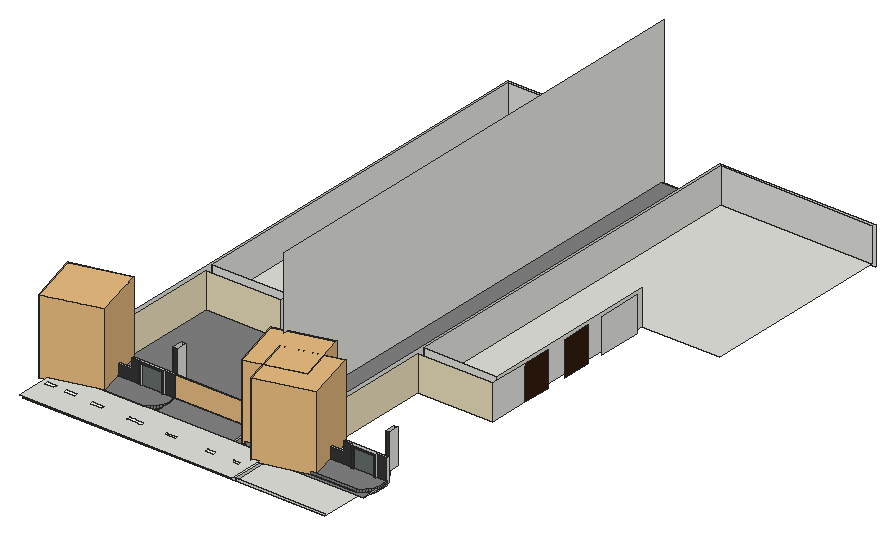
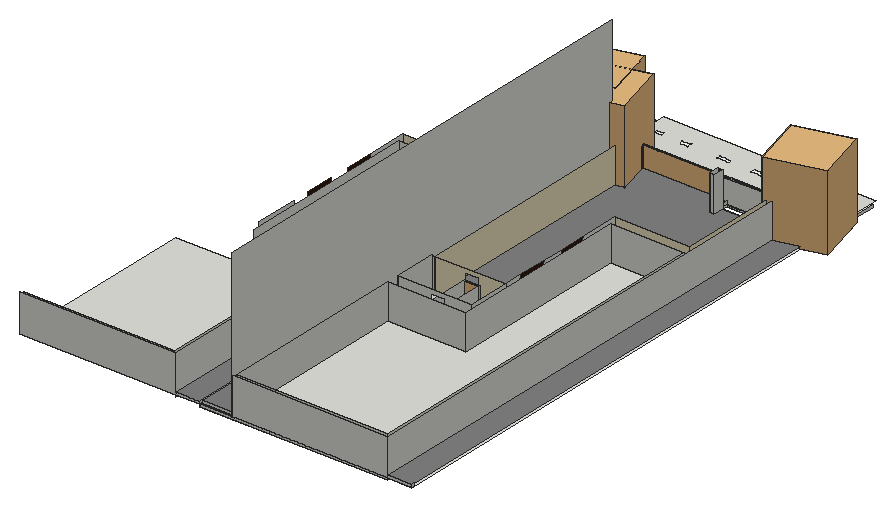
# SketchUp Ruby script. Lengths in inches.
U = 1.inch
M = Sketchup.active_model
def pt(a) = Geom::Point3d.new(a.map { |v| v * U })
def face(e, loops, mat)
  f = e.add_face(loops[0].map { |a| pt(a) })
  loops[1..].each { |l| e.add_face(l.map { |a| pt(a) }).erase! }
  f.material = f.back_material = mat if mat
  f
end
# faces: each face lists its corners as indices into pts; further lists are holes
def faces(e, pts, list, mat = nil) = list.each { |f| face(e, (f[0].is_a?(Array) ? f : [f]).map { |l| l.map { |i| pts[i] } }, mat) }
# xy, xz, yz: faces in a plane at the given z, y or x. An outline is a flat list of corners, or four numbers for a rectangle; further outlines are holes
def ring(l) = l.size == 4 ? [[l[0], l[1]], [l[2], l[1]], [l[2], l[3]], [l[0], l[3]]] : l.each_slice(2).to_a
def flat(e, list, mat, &to3) = list.each { |f| face(e, (f[0].is_a?(Array) ? f : [f]).map { |l| ring(l).map { |u, v| to3.(u, v) } }, mat) }
def xy(e, z, list, mat = nil) = flat(e, list, mat) { |x, y| [x, y, z] }
def xz(e, y, list, mat = nil) = flat(e, list, mat) { |x, z| [x, y, z] }
def yz(e, x, list, mat = nil) = flat(e, list, mat) { |y, z| [x, y, z] }
def lines(e, pts, list) = list.each { |a, b| e.add_line(pt(pts[a]), pt(pts[b])) }
# prism: a flat outline (further loops are holes) pulled along v
def prism(e, loops, v, mat = nil)
  f = face(e, loops, mat); d = Geom::Vector3d.new(v.map { |x| x * U })
  f.pushpull(f.normal.samedirection?(d) ? d.length : -d.length)
end
def box(e, o, s, mat = nil) = prism(e, [[o, [o[0] + s[0], o[1], o[2]], [o[0] + s[0], o[1] + s[1], o[2]], [o[0], o[1] + s[1], o[2]]]], [0, 0, s[2]], mat)
def at(x, y, z, deg = 0) = Geom::Transformation.translation(pt([x, y, z])) * Geom::Transformation.rotation(ORIGIN, Z_AXIS, deg.degrees)
def axes(o, x, y, z) = Geom::Transformation.new([*x, 0, *y, 0, *z, 0, *pt(o).to_a, 1])
def part(name) = M.definitions.add(name)
# library, detail: a bought-in or finely detailed component or shape, given as its bounding box
def library(name, o, s) = part(name).tap { |d| box(d.entities, o, s) }
def detail(e, o, s) = box(e.add_group.entities, o, s)
def put(e, d, t, mat = nil) = e.add_instance(d, t).tap { |i| i.material = mat if mat }
def group(e, t, mat = nil) = e.add_group.tap { |g| g.transformation = t; g.material = mat if mat }.entities
root = M.entities
M.materials.add("Color_000").color = [255, 255, 255]
M.materials.add("[Color D01]").color = [237, 225, 189]
M.materials.add("[Slate Light Tile]").color = [54, 54, 54]
M.materials.add("[Slate]").color = [102, 110, 108]
M.materials.add("[Tile Grey]").color = [130, 130, 130]
M.materials.add("[Wood Veneer 01]").color = [51, 28, 15]
c1 = library("Palm tree",[-4.09,-4.52,0],[193.52,193.51,258.93])
c2 = part("Palm+Tree")
put(c2.entities,c1,at(25.51,-21.81,0,15))
c3 = part("Untitled (5)")
xy(c3.entities,0,[[[158.81,26.5625,306.06,993.3125],[226.57,518.17,239.57,583.92],[225.28,357.51,237.28,411.51],[222.61,182.28,236.36,226.53],[239.71,931.55,251.46,972.3],[233.64,703.93,242.14,755.18],[240.05,835.03,248.8,880.53],[222.04,66.5,231.29,100.5]]])
xy(c3.entities,0,[[222.04,66.5,231.29,100.5],[222.61,182.28,236.36,226.53],[225.28,357.51,237.28,411.51],[226.57,518.17,239.57,583.92],[233.64,703.93,242.14,755.18],
  [240.05,835.03,248.8,880.53],[239.71,931.55,251.46,972.3]],"Color_000")
c4 = library("Sliding Gate",[0,0,0],[194.88,4.13,70.58])
c5 = library("元件\#5",[-4.39,0,0],[5.37,35.83,90.55])
xy(root,-6.875,[[0,14.47,0,159.14,302.45,159.14,309.52,163.79,310.12,164.29,310.12,14.47],[310.12,14.47,310.12,164.29,316.04,169.1875,321.92,175.27,327.11,181.96,331.52,189.18,335.11,196.84,337.76,204.6,337.76,246.64,310.12,246.64,310.12,294.84,603.24,294.84,603.24,14.47],[603.24,14.47,603.24,246.64,605.72,246.64,605.72,228.12,608.25,219.11,611.63,210.38,615.8125,202.01,620.77,194.08,626.45,186.64,632.81,179.78,639.78,173.54,647.32,167.99,655.34,163.18,663.79,159.14,733.5625,159.14,733.5625,14.47],[733.5625,14.47,733.5625,159.14,1036.01,159.14,1043.08,163.79,1043.68,164.29,1043.68,14.47],[0,159.14,0,164.29,310.12,164.29,309.52,163.79,302.45,159.14],
  [663.79,159.14,655.34,163.18,647.32,167.99,639.78,173.54,632.81,179.78,626.45,186.64,620.77,194.08,615.8125,202.01,611.63,210.38,608.25,219.11,605.72,228.12,605.72,246.64,733.5625,246.64,733.5625,159.14],[733.5625,159.14,733.5625,164.29,1043.68,164.29,1043.08,163.79,1036.01,159.14],[0,164.29,310.12,246.64],[310.12,164.29,310.12,246.64,337.76,246.64,337.76,204.6,335.11,196.84,331.52,189.18,327.11,181.96,321.92,175.27,316.04,169.1875],[733.5625,164.29,1043.68,246.64],
  [1043.68,164.29,1043.68,246.64,1071.32,246.64,1071.32,204.6,1068.68,196.84,1065.08,189.18,1060.67,181.96,1055.49,175.27,1049.6,169.1875],[83.125,246.64,83.125,2003.89,733.5625,2003.89,733.5625,246.64,603.24,246.64,603.24,294.84,101.95,294.84,101.95,255.71,310.12,255.71,310.12,246.64]])
xy(root,0,[[0,14.47,733.5625,146.33],[337.76,146.33,603.24,204.6],[603.24,146.33,605.72,204.6],[0,159.14,302.45,159.14,309.52,163.79,310.12,164.29,0,164.29],[663.79,159.14,733.5625,159.14,733.5625,204.6,614.52,204.6,615.8125,202.01,620.77,194.08,626.45,186.64,632.81,179.78,639.78,173.54,647.32,167.99,655.34,163.18],
  [733.5625,159.14,1036.01,159.14,1043.08,163.79,1043.68,164.29,733.5625,164.29],[0,164.29,310.12,246.64],[310.12,164.29,316.04,169.1875,321.92,175.27,327.11,181.96,331.52,189.18,335.11,196.84,337.76,204.6,337.76,246.64,310.12,246.64],[733.5625,164.29,1043.68,246.64],[1043.68,164.29,1049.6,169.1875,1055.49,175.27,1060.67,181.96,1065.08,189.18,1068.68,196.84,1071.32,204.6,1071.32,246.64,1043.68,246.64],
  [337.76,204.6,337.84,204.85,339.68,213.11,340.59,221.52,340.57,229.98,339.625,238.39,337.76,246.64],[337.76,204.6,603.24,204.6,603.24,246.64,337.76,246.64,339.625,238.39,340.57,229.98,340.59,221.52,339.68,213.11,337.84,204.85],[603.24,204.6,605.72,204.6,605.72,228.12,604.04,237.32,603.24,246.64],[614.52,204.6,733.5625,204.6,733.5625,246.64,605.72,246.64,605.72,228.12,608.25,219.11,611.63,210.38],[1071.32,204.6,1071.32,246.64,1073.1875,238.39,1074.14,229.98,1074.15,221.52,1073.24,213.11,1071.41,204.85],
  [1071.32,204.6,1071.41,204.85,1073.24,213.11,1074.15,221.52,1074.14,229.98,1073.1875,238.39,1071.32,246.64],[605.72,228.12,605.72,246.64,603.24,246.64,604.04,237.32],[0,246.64,83.125,2003.89],[83.125,246.64,310.12,246.64,310.12,255.71,101.95,255.71,101.95,294.84,603.24,294.84,603.24,246.64,622,246.64,622,2003.89,83.125,2003.89],[310.12,246.64,337.76,255.71],
  [337.76,246.64,603.24,246.64,603.24,294.84,310.12,294.84,310.12,255.71,337.76,255.71],[622,246.64,733.5625,1994.39],[733.5625,246.64,816.6875,2003.89],[1043.68,246.64,1071.32,255.71],[622,1994.39,733.5625,2003.89]])
xy(root,0,[[0,146.33,337.76,146.33,337.76,204.6,335.11,196.84,331.52,189.18,327.11,181.96,321.92,175.27,316.04,169.1875,310.12,164.29,309.52,163.79,302.45,159.14,0,159.14],[605.72,146.33,733.5625,146.33,733.5625,159.14,663.79,159.14,655.34,163.18,647.32,167.99,639.78,173.54,632.81,179.78,626.45,186.64,620.77,194.08,615.8125,202.01,614.52,204.6,605.72,204.6],[733.5625,146.33,1071.32,146.33,1071.32,204.6,1068.68,196.84,1065.08,189.18,1060.67,181.96,1055.49,175.27,1049.6,169.1875,1043.68,164.29,1043.08,163.79,1036.01,159.14,733.5625,159.14],[605.72,204.6,614.52,204.6,611.63,210.38,608.25,219.11,605.72,228.12]],"[Tile Grey]")
xy(root,8.6875,[[91.76,714.9,344.07,714.9,344.07,1340.4,613.36,1340.4,613.36,1995.26,91.76,1995.26],[825.32,714.9,1077.64,714.9,1077.64,1340.4,1346.93,1340.4,1346.93,1995.26,825.32,1995.26],[358.6875,1150.15,452.08,1298.96],[500.08,1150.15,613.36,1298.96]])
xy(root,8.6875,[[0,159.14,302.45,159.14,309.52,163.79,316.04,169.1875,321.92,175.27,327.11,181.96,331.52,189.18,335.11,196.84,337.84,204.85,339.68,213.11,340.59,221.52,340.57,229.98,339.625,238.39,337.76,246.64,303.85,246.64,303.85,243.46,295.95,243.46,295.95,246.64,224.55,246.64,224.55,243.46,215.84,243.46,215.84,246.64,83.125,246.64,83.125,2003.89,0,2003.89],[663.79,159.14,733.5625,159.14,733.5625,1994.39,622,1994.39,622,246.64,603.24,246.64,604.04,237.32,605.72,228.12,608.25,219.11,611.63,210.38,615.8125,202.01,620.77,194.08,626.45,186.64,632.81,179.78,639.78,173.54,647.32,167.99,655.34,163.18],[733.5625,159.14,1036.01,159.14,1043.08,163.79,1049.6,169.1875,1055.49,175.27,1060.67,181.96,1065.08,189.18,1068.68,196.84,1071.41,204.85,1073.24,213.11,1074.15,221.52,1074.14,229.98,1073.1875,238.39,1071.32,246.64,1037.42,246.64,1037.42,243.46,1029.51,243.46,1029.51,246.64,958.11,246.64,958.11,243.46,949.4,243.46,949.4,246.64,816.6875,246.64,816.6875,2003.89,733.5625,2003.89],[310.12,246.64,603.24,246.64,603.24,1150.15,500.08,1150.15,500.08,1298.96,452.08,1298.96,452.08,1150.15,358.6875,1150.15,358.6875,679.27,99.82,679.27,99.82,310.87,101.95,310.87,101.95,294.84,294.56,294.84,294.56,329.78,310.12,329.78]],"[Tile Grey]")
xz(root,14.47,[[0,-6.875,310.12,0],[310.12,-6.875,603.24,0],[603.24,-6.875,733.5625,0],[733.5625,-6.875,1043.68,0]])
xz(root,159.14,[[0,-6.875,302.45,0],[663.79,-6.875,733.5625,0],[733.5625,-6.875,1036.01,0]])
xz(root,159.14,[[0,0,302.45,8.6875],[663.79,0,733.5625,8.6875],[733.5625,0,1036.01,8.6875]],"[Tile Grey]")
xz(root,243.46,[[215.84,8.6875,224.55,8.6875,224.55,74.24,295.95,74.24,295.95,8.6875,303.85,8.6875,303.85,79.95,215.84,79.95],[949.4,8.6875,958.11,8.6875,958.11,74.24,1029.51,74.24,1029.51,8.6875,1037.42,8.6875,1037.42,79.95,949.4,79.95]],"[Slate Light Tile]")
xz(root,246.64,[[0,-6.875,83.125,0],[83.125,-6.875,310.12,0],[310.12,-6.875,337.76,0],[603.24,-6.875,605.72,0],[605.72,-6.875,733.5625,0],
  [733.5625,-6.875,816.6875,0],[816.6875,-6.875,1043.68,0],[1043.68,-6.875,1071.32,0],[310.12,0,337.76,8.6875],[337.76,0,603.24,8.6875],
  [603.24,0,605.72,8.6875],[1043.68,0,1071.32,8.6875]])
xz(root,246.64,[[83.125,8.6875,215.84,8.6875,215.84,79.95,188.54,79.95,188.54,44.76,115.73,44.76,115.73,79.95,83.125,79.95],[303.85,8.6875,337.76,79.95],[603.24,8.6875,622,76.4375],[816.6875,8.6875,949.4,8.6875,949.4,79.95,922.1,79.95,922.1,44.76,849.29,44.76,849.29,79.95,816.6875,79.95],[1037.42,8.6875,1071.32,79.95]],"[Slate Light Tile]")
xz(root,246.64,[[224.55,8.6875,295.95,74.24],[958.11,8.6875,1029.51,74.24]],"[Slate]")
xz(root,255.71,[[101.95,-6.875,310.12,0],[835.51,-6.875,1043.68,0],[101.95,0,101.95,79.95,115.73,79.95,115.73,44.76,188.54,44.76,188.54,79.95,337.76,79.95,337.76,0],[835.51,0,835.51,79.95,849.29,79.95,849.29,44.76,922.1,44.76,922.1,79.95,1071.32,79.95,1071.32,0]])
xz(root,294.84,[[101.95,-6.875,294.56,0],[294.56,-6.875,310.12,0],[310.12,-6.875,603.24,0],[835.51,-6.875,1028.12,0],[1028.12,-6.875,1043.68,0],
  [101.95,0,294.56,8.6875],[835.51,0,1028.12,8.6875]])
xz(root,294.84,[[294.56,0,310.12,128.6875],[1028.12,0,1043.68,128.6875]],"[Slate Light Tile]")
xz(root,310.87,[[99.82,8.6875,101.95,128.6875],[833.39,8.6875,835.51,128.6875]])
xz(root,329.78,[[294.56,8.6875,310.12,128.6875],[1028.12,8.6875,1043.68,128.6875]])
xz(root,679.27,[[99.82,8.6875,358.6875,128.6875],[833.39,8.6875,1092.25,128.6875]],"[Color D01]")
xz(root,714.9,[[91.76,8.6875,344.07,128.6875],[825.32,8.6875,1077.64,128.6875]])
xz(root,1150.15,[[603.24,8.6875,613.36,128.6875]])
xz(root,1150.15,[[358.6875,8.6875,452.08,8.6875,452.08,114.3125,500.08,114.3125,500.08,8.6875,603.24,8.6875,603.24,128.6875,358.6875,128.6875]],"[Color D01]")
xz(root,1298.96,[[358.6875,8.6875,358.6875,128.6875,613.36,128.6875,613.36,8.6875,500.08,8.6875,500.08,114.3125,452.08,114.3125,452.08,8.6875]])
xz(root,1340.4,[[344.07,8.6875,613.36,128.6875]])
xz(root,1994.39,[[622,0,733.5625,8.6875]])
xz(root,1995.26,[[91.76,8.6875,613.36,128.6875],[825.32,8.6875,1346.93,128.6875]])
xz(root,2003.89,[[83.125,-6.875,733.5625,0],[0,0,83.125,8.6875],[83.125,0,622,128.6875],[733.5625,0,816.6875,8.6875],[816.6875,0,1355.5625,128.6875]])
yz(root,0,[[14.47,-6.875,159.14,0],[159.14,-6.875,246.64,0],[1994.39,0,2003.89,8.6875]])
yz(root,83.125,[[246.64,-6.875,2003.89,0],[246.64,8.6875,246.64,79.95,286.21,79.95,286.21,120.375,293.46,120.375,293.46,128.6875,2003.89,128.6875,2003.89,8.6875]])
yz(root,91.76,[[714.9,8.6875,1995.26,128.6875]])
yz(root,99.82,[[310.87,8.6875,679.27,128.6875]],"[Color D01]")
yz(root,101.95,[[255.71,-6.875,286.21,0],[286.21,-6.875,294.84,0],[255.71,0,286.21,79.95]])
yz(root,101.95,[[286.21,0,294.84,0,294.84,8.6875,310.87,8.6875,310.87,128.6875,286.21,128.6875]],"[Slate Light Tile]")
yz(root,215.84,[[243.46,8.6875,246.64,79.95]])
yz(root,224.55,[[243.46,8.6875,246.64,74.24]])
yz(root,294.56,[[294.84,8.6875,329.78,128.6875]])
yz(root,295.95,[[243.46,8.6875,246.64,74.24]])
yz(root,303.85,[[243.46,8.6875,246.64,79.95]])
yz(root,310.12,[[246.64,-6.875,255.71,0],[255.71,-6.875,294.84,0],[246.64,0,294.84,8.6875],[294.84,8.6875,329.78,128.6875]])
yz(root,337.76,[[204.6,-6.875,246.64,0],[146.33,0,246.64,8.6875,246.64,0],[246.64,0,255.71,79.95]])
yz(root,344.07,[[714.9,8.6875,1340.4,128.6875]])
yz(root,358.6875,[[679.27,8.6875,818.04,128.6875],[914.71,8.6875,987.36,128.6875],[1088.15,8.6875,1150.15,128.6875],[1150.15,8.6875,1298.96,128.6875]])
yz(root,358.6875,[[818.04,8.6875,914.71,128.6875],[987.36,8.6875,1088.15,128.6875]],"[Wood Veneer 01]")
yz(root,452.08,[[1150.15,8.6875,1298.96,91.5625]])
yz(root,500.08,[[1150.15,8.6875,1298.96,91.5625]])
yz(root,603.24,[[246.64,-6.875,286.21,0],[286.21,-6.875,294.84,0],[246.64,0,286.21,8.6875],[286.21,0,294.84,8.6875]])
yz(root,603.24,[[316.26,8.6875,1150.15,128.6875]],"[Color D01]")
yz(root,603.24,[[246.64,8.6875,286.21,76.4375],[286.21,8.6875,316.26,128.6875]],"[Slate Light Tile]")
yz(root,605.72,[[228.12,-6.875,246.64,0],[146.33,0,228.12,0,228.12,7.08],[228.12,0,246.64,0,246.64,8.6875,228.12,7.08]])
yz(root,613.36,[[1150.15,8.6875,1298.96,128.6875],[1340.4,8.6875,1995.26,128.6875]])
yz(root,622,[[1994.39,0,2003.89,0,2003.89,506.6875,361.27,506.6875,361.27,154.75,266.43,154.75,266.43,140.625,246.64,140.625,246.64,120.375,286.21,120.375,286.21,76.4375,246.64,76.4375,246.64,8.6875,1994.39,8.6875]])
yz(root,733.5625,[[14.47,-6.875,159.14,0],[159.14,-6.875,246.64,0],[246.64,-6.875,2003.89,0],[159.14,0,1994.39,8.6875],[1994.39,0,2003.89,8.6875]])
yz(root,816.6875,[[246.64,-6.875,2003.89,0],[246.64,8.6875,246.64,79.95,286.21,79.95,286.21,120.375,293.46,120.375,293.46,128.6875,2003.89,128.6875,2003.89,8.6875]])
yz(root,825.32,[[714.9,8.6875,1995.26,128.6875]])
yz(root,833.39,[[310.87,8.6875,679.27,128.6875]],"[Color D01]")
yz(root,835.51,[[255.71,-6.875,286.21,0],[286.21,-6.875,294.84,0],[255.71,0,286.21,79.95]])
yz(root,835.51,[[286.21,0,294.84,0,294.84,8.6875,310.87,8.6875,310.87,128.6875,286.21,128.6875]],"[Slate Light Tile]")
yz(root,949.4,[[243.46,8.6875,246.64,79.95]])
yz(root,958.11,[[243.46,8.6875,246.64,74.24]])
yz(root,1028.12,[[294.84,8.6875,329.78,128.6875]])
yz(root,1029.51,[[243.46,8.6875,246.64,74.24]])
yz(root,1037.42,[[243.46,8.6875,246.64,79.95]])
yz(root,1043.68,[[246.64,-6.875,255.71,0],[255.71,-6.875,294.84,0],[246.64,0,294.84,8.6875],[294.84,8.6875,329.78,128.6875]])
yz(root,1071.32,[[204.6,-6.875,246.64,0],[146.33,0,246.64,8.6875,246.64,0],[246.64,0,255.71,79.95]])
yz(root,1077.64,[[714.9,8.6875,1340.4,128.6875]])
yz(root,1092.25,[[679.27,8.6875,818.04,128.6875],[1150.15,8.6875,1298.96,128.6875]])
yz(root,1092.25,[[818.04,8.6875,914.71,128.6875],[987.36,8.6875,1088.15,128.6875]],"[Wood Veneer 01]")
p = [[309.52,163.79,0],[302.45,159.14,0],[302.45,159.14,-6.875],[309.52,163.79,-6.875],[663.79,159.14,0],[655.34,163.18,0],
  [655.34,163.18,-6.875],[663.79,159.14,-6.875],[1043.08,163.79,0],[1036.01,159.14,0],[1036.01,159.14,-6.875],[1043.08,163.79,-6.875],
  [647.32,167.99,0],[647.32,167.99,-6.875],[316.04,169.1875,0],[310.12,164.29,0],[310.12,164.29,-6.875],[316.04,169.1875,-6.875],
  [1049.6,169.1875,0],[1043.68,164.29,0],[1043.68,164.29,-6.875],[1049.6,169.1875,-6.875],[639.78,173.54,0],[639.78,173.54,-6.875],
  [321.92,175.27,0],[321.92,175.27,-6.875],[1055.49,175.27,0],[1055.49,175.27,-6.875],[632.81,179.78,0],[632.81,179.78,-6.875],
  [327.11,181.96,0],[327.11,181.96,-6.875],[1060.67,181.96,0],[1060.67,181.96,-6.875],[626.45,186.64,0],[626.45,186.64,-6.875],
  [331.52,189.18,0],[331.52,189.18,-6.875],[1065.08,189.18,0],[1065.08,189.18,-6.875],[620.77,194.08,0],[620.77,194.08,-6.875],
  [335.11,196.84,0],[335.11,196.84,-6.875],[1068.68,196.84,0],[1068.68,196.84,-6.875],[615.8125,202.01,0],[615.8125,202.01,-6.875],
  [337.76,204.6,0],[337.76,204.6,-6.875],[1071.32,204.6,0],[1071.32,204.6,-6.875],[614.52,204.6,0],[611.63,210.38,0],
  [611.63,210.38,-6.875],[608.25,219.11,0],[608.25,219.11,-6.875],[605.72,228.12,0],[605.72,228.12,-6.875],[337.76,246.64,8.6875],
  [337.76,146.33,0],[603.24,146.33,0],[605.72,146.33,0],[605.72,228.12,7.08],[605.72,246.64,8.6875],[603.24,246.64,8.6875],
  [309.52,163.79,8.6875],[302.45,159.14,8.6875],[663.79,159.14,8.6875],[655.34,163.18,8.6875],[1043.08,163.79,8.6875],[1036.01,159.14,8.6875],
  [647.32,167.99,8.6875],[316.04,169.1875,8.6875],[1049.6,169.1875,8.6875],[639.78,173.54,8.6875],[321.92,175.27,8.6875],[1055.49,175.27,8.6875],
  [632.81,179.78,8.6875],[327.11,181.96,8.6875],[1060.67,181.96,8.6875],[626.45,186.64,8.6875],[331.52,189.18,8.6875],[1065.08,189.18,8.6875],
  [620.77,194.08,8.6875],[335.11,196.84,8.6875],[1068.68,196.84,8.6875],[615.8125,202.01,8.6875],[337.84,204.85,8.6875],[337.84,204.85,0],
  [1071.41,204.85,8.6875],[1071.41,204.85,0],[611.63,210.38,8.6875],[339.68,213.11,8.6875],[339.68,213.11,0],[1073.24,213.11,8.6875],
  [1073.24,213.11,0],[608.25,219.11,8.6875],[340.59,221.52,8.6875],[340.59,221.52,0],[1074.15,221.52,8.6875],[1074.15,221.52,0],
  [605.72,228.12,8.6875],[340.57,229.98,8.6875],[340.57,229.98,0],[1074.14,229.98,8.6875],[1074.14,229.98,0],[604.04,237.32,8.6875],
  [604.04,237.32,0],[339.625,238.39,8.6875],[339.625,238.39,0],[1073.1875,238.39,8.6875],[1073.1875,238.39,0],[603.24,246.64,0],
  [337.76,246.64,0],[1071.32,246.64,8.6875],[1071.32,246.64,0]]
faces(root,p,[[0,1,2,3],[4,5,6,7],[8,9,10,11],[5,12,13,6],[14,15,0,3,16,17],[18,19,8,11,20,21],[12,22,23,13],[24,14,17,25],
  [26,18,21,27],[22,28,29,23],[30,24,25,31],[32,26,27,33],[28,34,35,29],[36,30,31,37],[38,32,33,39],[34,40,41,35],
  [42,36,37,43],[44,38,39,45],[40,46,47,41],[48,42,43,49],[50,44,45,51],[52,53,54,47,46],[53,55,56,54],[55,57,58,56]])
faces(root,p,[[59,60,61,62,63,64,65],[66,67,1,0],[68,69,5,4],[70,71,9,8],[69,72,12,5],[73,66,0,15,14],[74,70,8,19,18],[72,75,22,12],
  [76,73,14,24],[77,74,18,26],[75,78,28,22],[79,76,24,30],[80,77,26,32],[78,81,34,28],[82,79,30,36],[83,80,32,38],
  [81,84,40,34],[85,82,36,42],[86,83,38,44],[84,87,46,40],[88,85,42,48,89],[90,86,44,50,91],[87,92,53,52,46],[93,88,89,94],
  [95,90,91,96],[92,97,55,53],[98,93,94,99],[100,95,96,101],[97,102,63,57,55],[103,98,99,104],[105,100,101,106],[102,107,108,57,63],
  [109,103,104,110],[111,105,106,112],[107,65,113,108],[59,109,110,114],[115,111,112,116]],"[Tile Grey]")
put(root,c2,at(-47.9375,141.91,0))
put(root,c3,axes([753.72,-171.64,8.6875],[0,1.08078,0],[-0.75879,0,0],[0,0,1]))
put(root,c4,axes([337.76,246.64,8.6875],[1.37,0,0],[0,1,0],[0,0,1]))
put(root,c5,axes([447.87,1151.01,-17.4375],[0,-0.89,0],[1.45734,0,0],[0,0,1.20374]))
put(root,c2,at(603.24,204.6,0))
put(root,c2,at(685.625,141.91,0))
